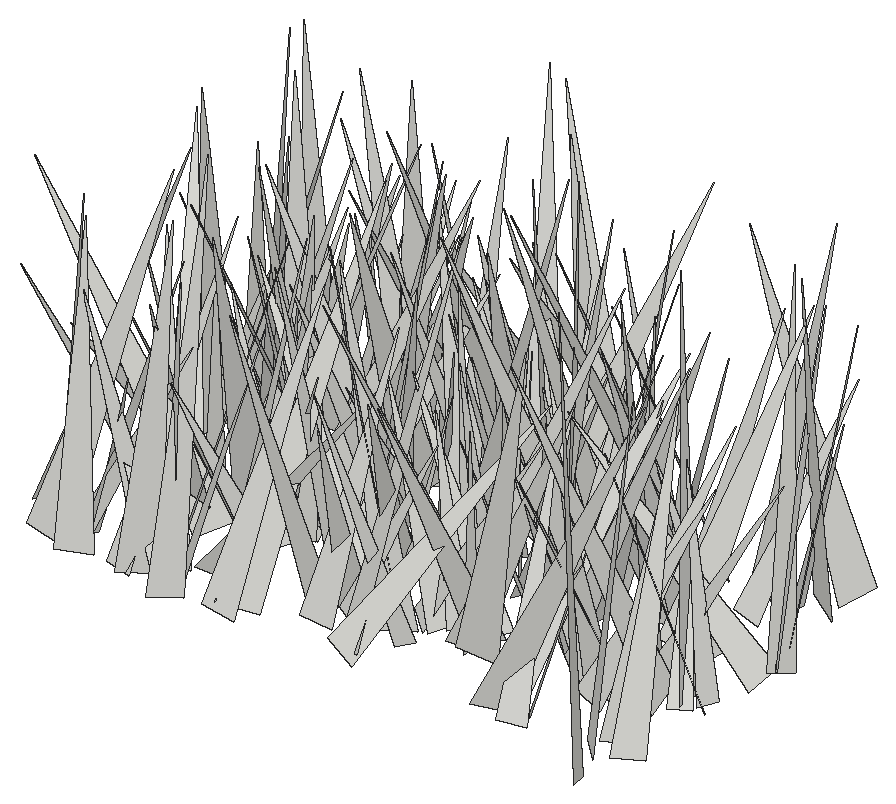
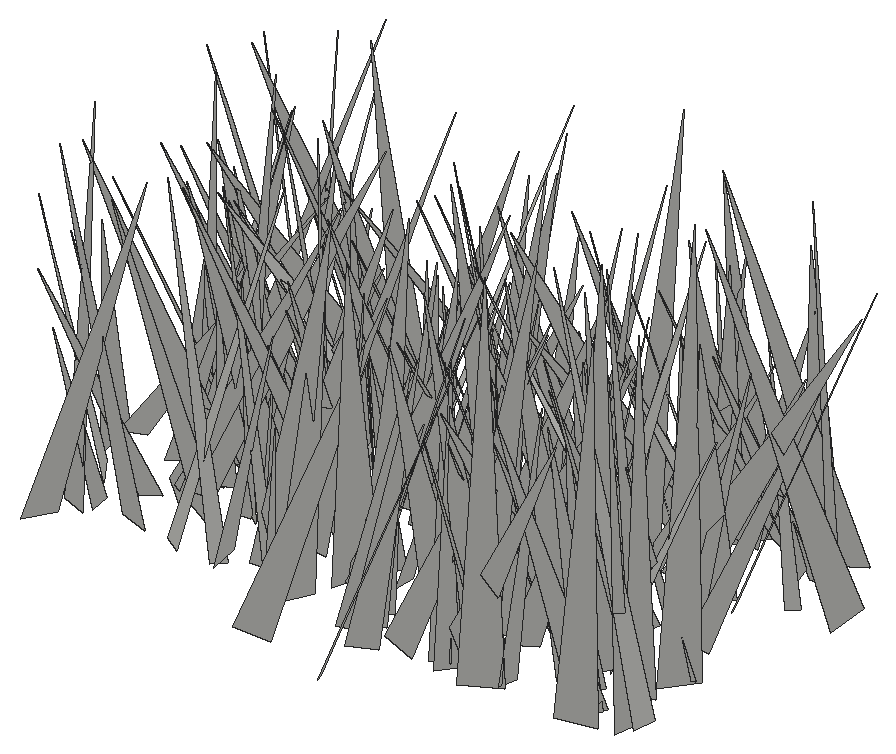
# SketchUp Ruby script. Lengths in inches.
U = 1.inch
M = Sketchup.active_model
def pt(a) = Geom::Point3d.new(a.map { |v| v * U })
def face(e, loops, mat)
  f = e.add_face(loops[0].map { |a| pt(a) })
  loops[1..].each { |l| e.add_face(l.map { |a| pt(a) }).erase! }
  f.material = f.back_material = mat if mat
  f
end
# faces: each face lists its corners as indices into pts; further lists are holes
def faces(e, pts, list, mat = nil) = list.each { |f| face(e, (f[0].is_a?(Array) ? f : [f]).map { |l| l.map { |i| pts[i] } }, mat) }
# xy, xz, yz: faces in a plane at the given z, y or x. An outline is a flat list of corners, or four numbers for a rectangle; further outlines are holes
def ring(l) = l.size == 4 ? [[l[0], l[1]], [l[2], l[1]], [l[2], l[3]], [l[0], l[3]]] : l.each_slice(2).to_a
def flat(e, list, mat, &to3) = list.each { |f| face(e, (f[0].is_a?(Array) ? f : [f]).map { |l| ring(l).map { |u, v| to3.(u, v) } }, mat) }
def xy(e, z, list, mat = nil) = flat(e, list, mat) { |x, y| [x, y, z] }
def xz(e, y, list, mat = nil) = flat(e, list, mat) { |x, z| [x, y, z] }
def yz(e, x, list, mat = nil) = flat(e, list, mat) { |y, z| [x, y, z] }
def lines(e, pts, list) = list.each { |a, b| e.add_line(pt(pts[a]), pt(pts[b])) }
# prism: a flat outline (further loops are holes) pulled along v
def prism(e, loops, v, mat = nil)
  f = face(e, loops, mat); d = Geom::Vector3d.new(v.map { |x| x * U })
  f.pushpull(f.normal.samedirection?(d) ? d.length : -d.length)
end
def box(e, o, s, mat = nil) = prism(e, [[o, [o[0] + s[0], o[1], o[2]], [o[0] + s[0], o[1] + s[1], o[2]], [o[0], o[1] + s[1], o[2]]]], [0, 0, s[2]], mat)
def at(x, y, z, deg = 0) = Geom::Transformation.translation(pt([x, y, z])) * Geom::Transformation.rotation(ORIGIN, Z_AXIS, deg.degrees)
def axes(o, x, y, z) = Geom::Transformation.new([*x, 0, *y, 0, *z, 0, *pt(o).to_a, 1])
def part(name) = M.definitions.add(name)
# library, detail: a bought-in or finely detailed component or shape, given as its bounding box
def library(name, o, s) = part(name).tap { |d| box(d.entities, o, s) }
def detail(e, o, s) = box(e.add_group.entities, o, s)
def put(e, d, t, mat = nil) = e.add_instance(d, t).tap { |i| i.material = mat if mat }
def group(e, t, mat = nil) = e.add_group.tap { |g| g.transformation = t; g.material = mat if mat }.entities
root = M.entities
c1 = part("fur_instance\#9")
p = [[0.8125,0,1.79],[0.67,-0.02,1.48],[0,-0.11,0],[0,0.11,0]]
faces(c1.entities,p,[[0,1,2,3]])
put(root,c1,axes([504.1,56.19,-21.86],[-7.32928,-2.99407,2.48715],[-3.76161,6.81126,-2.88543],[1.00033,3.67572,7.37273]))
put(root,c1,axes([480.44,57.9,-21.86],[-2.28357,5.70644,2.33564],[6.0895,2.47813,-0.10083],[0.96778,-2.12809,6.14557]))
put(root,c1,axes([483.11,58.11,-21.86],[4.75602,-4.66812,2.75377],[-5.20371,-4.95731,0.58378],[-1.51526,2.37234,6.63855]))
put(root,c1,axes([478.87,59.24,-21.86],[6.37942,2.61315,2.43113],[3.05762,-6.56979,-0.96169],[-1.84118,-1.85616,6.82648]))
put(root,c1,axes([483.21,58.84,-21.66],[0.69074,-4.72184,2.34998],[-4.89788,-1.45354,-1.48096],[-1.95676,1.97148,4.53648]))
put(root,c1,axes([503.06,58.16,-21.86],[4.54729,4.68314,2.12923],[4.88324,-4.82336,0.17985],[-1.61844,-1.39522,6.52513]))
put(root,c1,axes([484.17,58.3,-21.66],[-2.33068,3.85921,0.35584],[3.66264,2.05758,1.6744],[-1.26695,-1.15111,4.18592]))
put(root,c1,axes([479.25,57.9,-21.66],[0.24663,7.62872,2.41582],[7.70784,0.42293,-2.12242],[2.15005,-2.39126,7.33168]))
put(root,c1,axes([484.18,58.44,-21.86],[3.06348,4.37723,2.06786],[4.6001,-3.39453,0.37061],[-1.50841,-1.46222,5.32989]))
put(root,c1,axes([498.79,57.98,-21.66],[5.79439,-3.93356,1.43708],[-4.17619,-5.2444,2.48372],[0.31237,2.85246,6.54821]))
put(root,c1,axes([489.16,60.53,-21.86],[-5.96376,-1.66281,1.60864],[-1.32131,6.09893,1.40577],[1.89916,-0.97833,6.02952]))
put(root,c1,axes([490.28,61.08,-21.86],[3.42227,-3.49613,0.30492],[-3.40506,-3.41104,-0.89344],[-0.84941,-0.41195,4.81005]))
put(root,c1,axes([487.02,57.62,-21.86],[0.10942,6.44965,1.02032],[6.44115,0.06102,-1.07648],[1.07264,-1.02435,6.36012]))
put(root,c1,axes([495.81,61.57,-21.66],[2.24091,-5.47361,0.67385],[-5.23088,-2.33999,-1.61199],[-1.7471,-0.01469,5.69066]))
put(root,c1,axes([479.77,59.16,-21.86],[2.82226,4.09729,0.68802],[3.94816,-2.38599,-1.98631],[1.29353,-1.65697,4.56152]))
put(root,c1,axes([499.8,57.86,-21.86],[-1.60174,4.9541,0.61833],[4.97114,1.64265,-0.28364],[0.46172,-0.4996,5.19887]))
put(root,c1,axes([479.1,61.22,-21.86],[4.69242,0.16576,0.10905],[0.19618,-4.2622,-1.96297],[-0.02968,-1.96577,4.26532]))
put(root,c1,axes([484.67,58.49,-21.86],[3.7464,3.46532,0.67043],[3.46985,-3.79505,0.22613],[-0.64655,-0.28736,5.09832]))
put(root,c1,axes([499.99,63.17,-21.66],[-3.50557,-5.51536,0.11612],[-4.95597,3.20905,2.80393],[2.42302,-1.41579,5.90306]))
put(root,c1,axes([496.09,60.58,-21.66],[2.2039,-6.87435,1.74953],[-7.02125,-1.85328,1.56272],[1.00974,2.1174,7.04782]))
put(root,c1,axes([493.7,59.63,-21.66],[-0.77186,4.35622,1.72795],[4.2436,-0.09339,2.13104],[-1.98854,-1.8902,3.87699]))
put(root,c1,axes([503.06,62.18,-21.66],[-7.42684,-1.75978,1.28146],[-1.36577,7.3143,2.12899],[1.69519,-1.81689,7.32954]))
put(root,c1,axes([484.9,62.6,-21.66],[7.37439,-3.31849,1.28024],[-2.90244,-7.31769,-2.24953],[-2.05603,-1.57231,7.76747]))
put(root,c1,axes([480.76,62.38,-21.86],[-5.31145,-3.30369,0.30508],[-3.10318,5.15062,1.7494],[1.17379,-1.33255,6.00546]))
put(root,c1,axes([483.85,58.97,-21.86],[-3.36286,5.21282,1.50099],[5.38655,3.41774,0.19865],[0.64152,-1.37145,6.20023]))
put(root,c1,axes([497.47,60.89,-21.86],[3.7363,2.07589,0.22504],[1.88074,-3.14536,-2.2112],[0.90706,-2.02911,3.65784]))
put(root,c1,axes([492.25,57.82,-21.66],[0.90469,6.24799,0.05202],[5.52251,-0.775,-2.9597],[2.92267,-0.46962,5.57638]))
put(root,c1,axes([485.13,57.0625,-21.66],[-7.34828,2.49323,1.09592],[2.03506,7.1224,-2.5582],[1.80991,2.11416,7.32591]))
put(root,c1,axes([482.32,62.46,-21.86],[0.60186,-6.09784,0.10298],[-6.0697,-0.58883,0.60707],[0.59415,0.16161,6.09732]))
put(root,c1,axes([485.96,61.68,-21.86],[-4.12735,0.23871,1.0618],[0.66209,3.85593,1.70672],[0.86374,-1.81501,3.76552]))
put(root,c1,axes([490.9,59.92,-21.66],[1.63148,3.88333,0.8996],[3.80186,-1.22375,-1.61232],[1.19808,-1.40479,3.89132]))
put(root,c1,axes([490.08,59.21,-21.86],[-0.68675,5.73435,1.62653],[5.78722,1.03346,-1.2],[1.42703,-1.4315,5.64928]))
put(root,c1,axes([490.99,63,-21.66],[5.45875,-2.61976,0.1584],[-2.41646,-5.15945,-2.05595],[-1.02417,-1.78972,5.6951]))
put(root,c1,axes([494.09,63.34,-21.66],[-5.79035,-4.99721,0.36352],[-4.82955,5.71454,1.62848],[1.33407,-1.00217,7.47317]))
put(root,c1,axes([500.6,61.71,-21.86],[4.51587,-1.82573,1.61231],[-1.49442,-4.75873,-1.20297],[-1.92343,-0.58918,4.72009]))
put(root,c1,axes([482.36,57.92,-21.86],[2.22729,6.28936,0.04999],[6.2767,-2.22605,0.40869],[-0.40191,0.08939,6.65956]))
put(root,c1,axes([492.16,61.09,-21.86],[4.02018,4.80904,4.066],[5.52928,-5.00439,0.45193],[-3.01434,-2.76593,6.25176]))
put(root,c1,axes([495.41,60.79,-21.66],[3.73995,-4.97965,1.07609],[-4.97131,-3.27521,2.12161],[1.114,2.10195,5.85517]))
put(root,c1,axes([486.33,59.02,-21.86],[4.06792,5.19434,1.22411],[5.14399,-4.22635,0.83955],[-1.42088,-0.42943,6.54403]))
put(root,c1,axes([492.65,60.54,-21.86],[0.55965,-6.1533,3.26603],[-6.71098,-1.35523,-1.40332],[-1.86889,3.02383,6.01722]))
put(root,c1,axes([480.29,58.99,-21.66],[4.99403,0.89918,1.35491],[0.3935,-4.91429,1.81096],[-1.5778,1.62046,4.74018]))
put(root,c1,axes([485.15,59.38,-21.66],[4.61387,-2.10989,0.31356],[-1.93342,-3.82099,2.73855],[0.90102,2.60502,4.2708]))
put(root,c1,axes([504.49,58.43,-21.86],[-5.42402,3.35952,0.54018],[3.08821,5.28712,-1.87283],[1.42868,1.32596,6.09909]))
put(root,c1,axes([498.83,62.82,-21.86],[1.2889,-4.23263,0.01136],[-4.22076,-1.28617,-0.32791],[-0.31699,-0.08469,4.41236]))
put(root,c1,axes([503.36,59.02,-21.86],[-4.3486,2.21974,0.80785],[1.83051,4.23636,-1.78683],[1.49303,1.27131,4.54366]))
put(root,c1,axes([495.49,61.08,-21.86],[-3.94466,-0.14605,1.57067],[-0.23954,4.23653,-0.20765],[1.55915,0.28136,3.94189]))
put(root,c1,axes([504.04,63.01,-21.86],[-3.65311,-4.50937,0.62916],[-4.48426,3.70309,0.50402],[0.78847,0.16789,5.78149]))
put(root,c1,axes([484.62,62.13,-21.66],[-2.52034,-4.28654,0.32351],[-4.12689,2.30776,-1.57296],[-1.20326,1.06349,4.71724]))
put(root,c1,axes([500.8125,60.82,-21.86],[0.87918,5.14411,1.43079],[4.85097,-0.16366,-2.39235],[2.23095,-1.67133,4.63805]))
put(root,c1,axes([500.65,61.4,-21.86],[-0.27177,-3.75184,1.87256],[-3.70908,-0.66019,-1.86105],[-1.95589,1.77327,3.26904]))
put(root,c1,axes([492.36,58.14,-21.66],[3.62911,6.60842,0.2466],[6.35712,-3.56375,1.94657],[-1.82181,0.72867,7.28371]))
put(root,c1,axes([477.17,60.625,-21.86],[7.79072,-0.23447,0.87822],[-0.35324,-7.76347,1.06082],[-0.83754,1.09323,7.72172]))
put(root,c1,axes([488.57,62.52,-21.86],[-6.02473,-0.71032,1.74625],[-0.51818,6.24626,0.75302],[1.81257,-0.57532,6.01954]))
put(root,c1,axes([483.25,62.12,-21.86],[-4.16636,5.9481,1.52453],[5.74666,3.12806,3.50054],[-2.16332,-3.14611,6.36276]))
put(root,c1,axes([493.76,61.55,-21.86],[-4.44101,1.77663,0.66677],[1.83519,4.45274,0.3588],[0.48276,-0.58331,4.76973]))
put(root,c1,axes([498.64,58.67,-21.86],[-2.65177,6.66161,0.65253],[5.97681,2.67255,-2.995],[3.01341,0.56142,6.51452]))
put(root,c1,axes([492.76,61.55,-21.86],[2.95433,4.07724,0.35212],[3.82019,-2.59183,-2.04072],[1.46767,-1.46099,4.60298]))
put(root,c1,axes([485.59,62.22,-21.86],[4.21997,-0.6182,0.41958],[-0.60999,-4.24047,-0.11271],[-0.43142,-0.05127,4.26352]))
put(root,c1,axes([496.74,62.95,-21.86],[5.27182,0.13194,1.25121],[0.40362,-5.28245,-1.14356],[-1.19165,-1.2055,5.14798]))
put(root,c1,axes([487.34,58.3,-21.86],[-5.76444,5.45156,1.05869],[4.71185,5.60881,-3.22628],[2.93919,1.70025,7.24841]))
put(root,c1,axes([494.29,61.92,-21.86],[-2.34318,3.21724,1.23905],[3.43189,2.31946,0.46753],[0.3286,-1.2829,3.95253]))
put(root,c1,axes([483.73,59.32,-21.86],[4.88269,3.53574,0.69101],[3.04894,-4.67553,2.3797],[-1.91908,1.56767,5.53887]))
put(root,c1,axes([498.39,62.54,-21.66],[4.54413,5.8348,1.67226],[5.93472,-3.83302,-2.75273],[1.27295,-2.95864,6.86415]))
put(root,c1,axes([479.79,65.66,-21.66],[4.40481,-2.70951,0.82389],[-1.71706,-3.76665,-3.20728],[-2.2521,-2.42766,4.05674]))
put(root,c1,axes([495.58,62.41,-21.86],[-3.16425,3.77948,0.90882],[3.82647,2.82214,1.58634],[-0.68447,-1.69527,4.66695]))
put(root,c1,axes([501.33,61.07,-21.66],[0.65579,5.75921,0.77226],[5.58682,-0.41126,-1.67728],[1.5976,-0.92592,5.54845]))
put(root,c1,axes([482.58,63.01,-21.86],[4.66089,-0.94094,1.87831],[-0.93791,-5.02216,-0.1885],[-1.87983,0.17273,4.75118]))
put(root,c1,axes([491.84,61.29,-21.86],[2.15657,3.40289,0.33157],[3.29952,-2.17412,0.8525],[-0.89598,0.18416,3.93747]))
put(root,c1,axes([485.83,62.66,-21.86],[-4.37438,2.14658,0.79892],[2.22863,4.38643,0.41683],[0.52851,-0.72986,4.85482]))
put(root,c1,axes([498.67,59.9375,-21.86],[4.76717,4.34009,0.09976],[4.0907,-4.54047,2.05487],[-1.45344,1.45601,6.11063]))
put(root,c1,axes([496.86,63.15,-21.86],[-3.19994,-2.12817,0.10035],[-2.08753,3.09569,-0.91527],[-0.42587,0.81635,3.73243]))
put(root,c1,axes([494.23,61.85,-21.66],[3.12045,6.97557,0.92804],[6.87353,-2.80376,-2.03727],[1.5081,-1.6545,7.36514]))
put(root,c1,axes([500.16,58.4375,-21.66],[5.94606,5.36025,0.59468],[4.2161,-5.17199,4.4628],[-3.36309,2.9933,6.64615]))
put(root,c1,axes([486.17,63.41,-21.86],[2.50338,-2.82714,1.30611],[-3.05988,-2.54469,0.35667],[-0.57944,1.22368,3.75931]))
put(root,c1,axes([481.11,64.24,-21.86],[-1.67954,-4.60165,1.09216],[-4.72861,1.65608,-0.29411],[0.09072,1.12742,4.88974]))
put(root,c1,axes([486.01,64.34,-21.86],[-1.02707,-3.52995,0.46815],[-3.49734,0.90838,-0.82343],[-0.66956,0.66999,3.58293]))
put(root,c1,axes([493.96,63.96,-21.86],[0.28904,-4.61969,1.68996],[-4.89331,-0.44312,-0.3744],[-0.50298,1.65624,4.61355]))
put(root,c1,axes([503.72,62.26,-21.86],[-2.57238,2.98987,0.10946],[2.97729,2.57237,-0.29516],[0.29502,0.10983,3.93311]))
put(root,c1,axes([490.69,65.67,-21.86],[1.56687,-4.2825,0.24372],[-4.04586,-1.5617,-1.43053],[-1.42486,-0.27491,4.32996]))
put(root,c1,axes([489.04,62.95,-21.66],[-3.06534,4.86368,0.18481],[4.51167,2.75744,2.26433],[-1.82603,-1.35165,5.28436]))
put(root,c1,axes([504.25,63.14,-21.86],[-4.36363,0.98227,0.81119],[0.91976,4.432,-0.41906],[0.88144,0.23814,4.45315]))
put(root,c1,axes([489.42,62.61,-21.86],[5.30824,4.83924,1.79848],[4.88732,-5.54151,0.48577],[-1.6634,-0.83881,7.16657]))
put(root,c1,axes([489.14,65.14,-21.86],[0.61294,-5.47928,1.38132],[-5.30961,-1.0339,-1.7451],[-1.93355,1.10218,5.22999]))
put(root,c1,axes([494.61,62.23,-21.66],[1.00631,5.78428,1.17144],[5.41169,-1.37849,2.15781],[-2.35451,-0.6962,5.46025]))
put(root,c1,axes([504.66,65.7,-21.86],[-5.96221,1.49508,0.02596],[1.36332,5.39133,2.61894],[-0.61423,-2.54602,5.56097]))
put(root,c1,axes([501.52,63.6875,-21.86],[3.29682,4.04593,0.27696],[3.82738,-2.98619,-1.93627],[1.34069,-1.42422,4.84659]))
put(root,c1,axes([503.54,63,-21.86],[-7.33304,-1.55705,2.53328],[-2.07568,7.50758,-1.39398],[2.1292,1.95633,7.36578]))
put(root,c1,axes([496.47,66.49,-21.66],[-7.7703,-1.5883,1.42664],[-1.2052,7.70803,2.01725],[1.76224,-1.7318,7.67014]))
put(root,c1,axes([499.97,65.46,-21.86],[-3.27673,-6.38483,2.25273],[-6.55108,3.62196,0.73666],[1.71005,1.64109,7.13865]))
put(root,c1,axes([488.47,65.77,-21.86],[6.1777,-0.38175,1.16241],[-0.13775,-6.16226,-1.29169],[-1.21571,-1.24165,6.0532]))
put(root,c1,axes([500.65,66.79,-21.86],[1.25653,-6.81976,0.6894],[-6.81087,-1.32116,-0.65555],[-0.77223,0.55558,6.90349]))
put(root,c1,axes([481.75,62.23,-21.86],[-3.35316,6.39569,0.22234],[6.39729,3.34326,0.30873],[-0.17041,-0.34016,7.2148]))
put(root,c1,axes([483.33,65.99,-21.66],[0.81031,-5.69395,0.84212],[-5.55553,-0.55126,1.61834],[1.50543,1.03047,5.51893]))
put(root,c1,axes([484.76,65.59,-21.86],[-4.52954,-3.25843,1.35312],[-3.24257,4.71245,0.49358],[1.39071,0.3748,5.55792]))
put(root,c1,axes([482.9375,68.11,-21.86],[-3.5223,-6.70382,0.02091],[-6.50166,3.42181,1.83516],[1.63401,-0.83562,7.34711]))
put(root,c1,axes([497.63,65.5,-21.86],[5.75538,-1.33671,0.29214],[-1.31847,-5.75568,-0.36093],[-0.36579,-0.28603,5.89753]))
put(root,c1,axes([488.43,63.11,-21.86],[-0.08905,4.06249,0.07241],[4.03019,0.09752,-0.5148],[0.51634,-0.06053,4.03072]))
put(root,c1,axes([484.27,66.37,-21.66],[6.50516,0.09741,3.11354],[0.81371,-7.01185,-1.48071],[-3.00691,-1.68675,6.33514]))
put(root,c1,axes([488.26,64.5,-21.86],[6.38411,4.40631,2.11358],[4.61615,-6.57865,-0.22824],[-1.60436,-1.39477,7.75373]))
put(root,c1,axes([489.65,66.72,-21.86],[4.97524,0.71585,1.07536],[1.04452,-4.74693,-1.67259],[-0.76015,-1.83742,4.74004]))
put(root,c1,axes([487.48,68.32,-21.66],[7.10031,-2.91459,1.55919],[-2.29482,-7.00551,-2.64516],[-2.37902,-1.94118,7.20502]))
put(root,c1,axes([502.35,66.26,-21.86],[-3.89042,0.9571,1.21715],[1.27935,3.84105,1.06884],[0.87221,-1.36496,3.86121]))
put(root,c1,axes([485.47,64.31,-21.86],[2.59444,7.48207,1.23534],[7.31718,-2.12705,-2.48457],[1.99156,-1.93206,7.51927]))
put(root,c1,axes([492.47,67.1875,-21.86],[1.67975,-3.93598,0.16611],[-3.93538,-1.66827,0.26597],[0.17974,0.25696,4.27115]))
put(root,c1,axes([492.36,64.86,-21.86],[-1.21025,6.4146,1.42422],[6.45546,0.89059,1.47445],[-1.22575,-1.64315,6.35907]))
put(root,c1,axes([478.85,67.82,-21.86],[7.55718,-3.05255,1.8054],[-2.7949,-7.74218,-1.39129],[-2.18313,-0.65505,8.03077]))
put(root,c1,axes([484.01,63.5,-21.86],[5.80303,5.01805,0.27093],[4.96083,-5.78629,0.91567],[-0.80277,0.51711,7.61693]))
put(root,c1,axes([499.78,66.62,-21.86],[0.85171,-3.4207,0.8533],[-3.50883,-0.73716,0.54719],[0.34265,0.95401,3.48241]))
put(root,c1,axes([497.82,68.2,-21.66],[3.38324,-1.277,0.34003],[-0.90165,-2.91389,-1.97203],[-0.96612,-1.75247,3.03119]))
put(root,c1,axes([493.62,66.04,-21.86],[3.14318,2.78213,1.66083],[2.96777,-3.40061,0.07991],[-1.30037,-1.03624,4.19683]))
put(root,c1,axes([495.13,65.65,-21.86],[4.37398,5.97616,2.1686],[6.29129,-4.44766,-0.43255],[-0.91492,-2.01317,7.39318]))
put(root,c1,axes([494.39,65.0625,-21.86],[4.56042,0.58445,0.815],[0.35248,-4.48653,1.24501],[-0.93891,1.15443,4.42595]))
put(root,c1,axes([492.39,67.45,-21.86],[-4.23671,-2.59002,0.97553],[-2.55905,4.34534,0.42292],[1.0541,0.13924,4.94763]))
put(root,c1,axes([496.08,65.73,-21.86],[-6.60957,-3.13791,3.29203],[-3.79035,7.01015,-0.92809],[2.51341,2.31982,7.25752]))
put(root,c1,axes([488.46,65.34,-21.66],[-5.41908,-0.82486,1.13145],[-1.12996,5.24719,-1.58656],[0.82691,1.76453,5.24687]))
put(root,c1,axes([490.73,68.125,-21.86],[-5.81258,-1.56867,1.18702],[-1.32265,5.85738,1.26392],[1.45614,-0.94136,5.88637]))
put(root,c1,axes([492.32,64.11,-21.86],[7.12046,1.58475,2.39098],[0.70942,-7.17277,2.64146],[-2.77938,2.22916,6.79964]))
put(root,c1,axes([495.375,67.24,-21.86],[-0.82021,3.34867,1.94688],[3.86928,0.61559,0.57127],[-0.18046,-2.02092,3.4]))
put(root,c1,axes([500.09,68.32,-21.86],[-2.49506,-7.82927,1.12782],[-7.54738,2.00233,-2.79687],[-2.3678,1.86761,7.7266]))
put(root,c1,axes([486.38,65.64,-21.86],[1.81357,5.35205,0.20733],[5.12174,-1.66889,-1.72019],[1.56691,-0.73948,5.38279]))
put(root,c1,axes([481.94,65.89,-21.66],[4.14579,-2.60609,2.17076],[-3.31381,-3.84297,1.71517],[-0.72292,2.67047,4.58667]))
put(root,c1,axes([485.58,68.54,-21.86],[5.39011,-5.98506,0.75501],[-6.02641,-5.29691,1.03406],[0.27067,1.25142,7.9878]))
put(root,c1,axes([500.95,65.53,-21.86],[-0.63507,6.95916,1.46669],[6.78735,1.03289,-1.962],[2.12438,-1.21968,6.70699]))
put(root,c1,axes([496.51,67.33,-21.86],[5.13759,-3.83835,0.8309],[-3.9202,-4.93031,1.46363],[0.23526,1.66651,6.24384]))
put(root,c1,axes([496.17,65.55,-21.86],[0.66695,4.37993,0.08385],[4.36286,-0.67176,0.3871],[-0.39533,-0.02429,4.41347]))
put(root,c1,axes([487.66,67.42,-21.86],[-2.49049,-3.07283,1.62396],[-3.33154,2.67981,-0.03854],[0.99012,1.28779,3.95516]))
put(root,c1,axes([481.58,68.15,-21.86],[3.73813,0.01426,0.67221],[0.17612,-3.68545,-0.90117],[-0.64889,-0.91811,3.62791]))
put(root,c1,axes([478.83,67.34,-21.86],[-0.2038,-3.57727,1.86557],[-3.68837,0.92217,1.36537],[1.63497,1.63446,3.31273]))
put(root,c1,axes([481.68,68.13,-21.86],[-3.75562,-3.58045,0.3486],[-3.58145,3.67402,-0.84892],[-0.33818,0.85312,5.11895]))
put(root,c1,axes([491.55,67.61,-21.86],[1.31397,-3.56018,1.31098],[-3.78942,-1.16427,0.63629],[0.18405,1.44556,3.7412]))
put(root,c1,axes([482.19,66.04,-21.66],[-7.10447,-2.39928,3.44832],[-3.25719,7.42464,-1.54476],[2.65295,2.69055,7.33783]))
put(root,c1,axes([500.8,68.17,-21.86],[-4.44374,-5.75342,0.61079],[-5.6055,4.0905,-2.25122],[-1.43294,1.84058,6.91236]))
put(root,c1,axes([486.62,68.15,-21.86],[3.50873,2.55931,1.93983],[3.03472,-3.58228,-0.76287],[-1.05048,-1.80039,4.27543]))
put(root,c1,axes([495.82,68.56,-21.66],[-1.13695,-6.80591,1.9758],[-6.92615,0.64332,-1.76957],[-1.50086,2.18691,6.66945]))
put(root,c1,axes([481.59,68.6875,-21.86],[3.84963,-3.94903,0.87916],[-4.01863,-3.87266,0.20133],[-0.4673,0.77142,5.51126]))
put(root,c1,axes([482.33,68.06,-21.86],[4.03772,-5.94106,3.0996],[-6.44975,-4.42725,-0.08397],[-1.8178,2.512,7.18278]))
put(root,c1,axes([490.3125,70.33,-21.86],[2.21636,-6.61774,0.25451],[-6.61771,-2.20273,0.35418],[0.25535,0.35358,6.97003]))
put(root,c1,axes([496.16,69.27,-21.86],[-2.04339,-2.88899,0.9747],[-2.5158,2.26047,1.42575],[1.7225,-0.12566,3.23866]))
put(root,c1,axes([494.73,65.73,-21.86],[-0.48607,6.36101,0.33267],[6.36907,0.48063,0.1158],[-0.09028,-0.34048,6.37851]))
put(root,c1,axes([479.46,69.23,-21.86],[0.11264,-6.37998,1.60761],[-6.5012,0.13924,1.0081],[1.01142,1.60553,6.30084]))
put(root,c1,axes([492.01,69.48,-21.86],[-2.55131,-7.67351,1.38924],[-7.65133,2.18082,-2.00574],[-1.50657,1.91917,7.83383]))
put(root,c1,axes([484.58,69.28,-21.66],[-5.48359,2.23586,1.70204],[2.68404,5.27249,1.72124],[0.83185,-2.27324,5.66623]))
put(root,c1,axes([484.99,67.45,-21.86],[3.70587,4.25797,0.60198],[4.28884,-3.60158,-0.92773],[0.31394,-1.06043,5.56805]))
put(root,c1,axes([497.92,67.63,-21.86],[2.53366,4.26731,1.78001],[4.34271,-2.89305,0.75426],[-1.5872,-1.10369,4.90515]))
put(root,c1,axes([484.93,66.3,-21.86],[-4.41851,1.16155,1.66424],[0.34777,4.36157,-2.12081],[1.99949,1.8082,4.04655]))
put(root,c1,axes([498.7,70.98,-21.86],[-4.09518,-5.32392,0.52178],[-5.17841,4.11019,1.29512],[1.34181,-0.38619,6.5907]))
put(root,c1,axes([481.69,69.83,-21.66],[3.71453,-6.09838,0.78607],[-6.05056,-3.46164,1.73599],[1.09493,1.55972,6.92635]))
put(root,c1,axes([486.46,67.35,-21.86],[1.13394,4.06883,0.24777],[4.07369,-1.14042,0.08414],[-0.14769,-0.216,4.22305]))
put(root,c1,axes([480.25,68.5,-21.86],[3.54049,4.95211,1.34575],[5.12044,-3.30078,-1.32493],[0.33991,-1.85767,5.94164]))
put(root,c1,axes([492.1,67.57,-21.66],[-6.74391,-2.32387,0.77011],[-2.44649,6.31426,-2.37034],[-0.09,2.49068,6.72772]))
put(root,c1,axes([496.625,71.03,-21.86],[6.71484,1.18998,0.43364],[1.2609,-6.06064,-2.89345],[0.11927,-2.92333,6.1752]))
put(root,c1,axes([493.99,67.27,-21.86],[-6.04222,-2.58238,2.07365],[-3.21518,5.60869,-2.38377],[0.79453,3.05796,6.1233]))
put(root,c1,axes([486.43,65.71,-21.66],[-4.56686,4.07542,0.09193],[3.68922,4.19072,-2.51023],[1.73411,1.8173,5.58247]))
put(root,c1,axes([486.96,69.03,-21.86],[1.79805,-6.87497,3.712],[-7.43664,-2.674,-1.35027],[-2.39594,3.14033,6.97674]))
put(root,c1,axes([504.51,66.375,-21.86],[3.51213,5.3509,1.08193],[4.75447,-3.63032,2.52063],[-2.68285,0.57134,5.88334]))
put(root,c1,axes([499.46,68.2,-21.86],[1.23681,5.98503,1.54047],[6.1022,-0.934,-1.27052],[0.97821,-1.7408,5.97797]))
put(root,c1,axes([504.84,66.48,-21.86],[-7.06937,0.92542,0.80535],[0.55425,6.6114,-2.73188],[1.09444,2.62944,6.58553]))
put(root,c1,axes([494.6,68.53,-21.66],[-1.73609,5.26171,0.91511],[5.1615,1.40586,1.70864],[-1.37182,-1.3693,5.27069]))
put(root,c1,axes([481.01,70.01,-21.86],[3.21186,-3.52218,0.8528],[-3.62385,-3.13,0.72104],[-0.02677,1.11644,4.71189]))
put(root,c1,axes([480.06,71.27,-21.86],[0.93957,-4.99379,0.05949],[-4.70596,-0.86502,1.71172],[1.67197,0.37157,4.78443]))
put(root,c1,axes([477.8125,71.03,-21.66],[8.03575,1.73258,0.69022],[1.85682,-7.7181,-2.24381],[-0.17451,-2.34107,7.90825]))
put(root,c1,axes([488.09,71.76,-21.86],[-1.10699,-6.38687,0.31821],[-6.26084,1.01671,-1.37367],[-1.30201,0.54128,6.33487]))
put(root,c1,axes([503.73,68.4,-21.86],[-4.45958,-2.36263,3.46386],[-3.3219,5.07642,-0.81428],[2.55838,2.47306,4.98064]))
put(root,c1,axes([503.09,70.93,-21.86],[-3.13728,-6.42445,2.27927],[-6.51063,3.56742,1.09378],[2.01998,1.52023,7.06539]))
put(root,c1,axes([492,69.18,-21.86],[-1.66543,4.2087,0.7623],[4.0491,1.28782,1.73616],[-1.37806,-1.30242,4.18002]))
put(root,c1,axes([492.68,68.1,-21.66],[1.48421,7.77893,1.22221],[7.56365,-1.06243,-2.42301],[2.19017,-1.60247,7.53948]))
put(root,c1,axes([484.43,71.35,-21.66],[3.61715,-5.66391,0.01487],[-5.50634,-3.51236,1.58351],[1.3268,0.86448,6.53117]))
put(root,c1,axes([486.34,71.6875,-21.86],[-0.53016,-5.209,0.61736],[-4.97847,0.69512,1.58982],[1.65216,0.4231,4.98871]))
put(root,c1,axes([489.72,67.49,-21.66],[-6.30964,2.41528,1.06239],[1.96226,6.1361,-2.29599],[1.76402,1.81341,6.35402]))
put(root,c1,axes([501.46,68.75,-21.86],[0.30593,5.01742,0.69432],[4.86404,-0.09691,-1.44288],[1.4134,-0.75252,4.8152]))
put(root,c1,axes([478.36,71.48,-21.86],[6.10646,0.88523,1.50787],[1.27518,-6.00248,-1.64024],[-1.19633,-1.87958,5.94829]))
put(root,c1,axes([483.56,71.375,-21.86],[4.6906,-0.13116,1.94102],[0.35682,-4.92253,-1.19491],[-1.91244,-1.24013,4.53774]))
put(root,c1,axes([485.85,71.95,-21.86],[5.31663,-1.02418,0.76649],[-0.77202,-5.18142,-1.56841],[-1.02002,-1.41668,5.18224]))
put(root,c1,axes([494.09,71.22,-21.86],[6.71325,2.37054,1.67819],[2.73448,-6.58312,-1.63968],[-0.97898,-2.13225,6.9281]))
put(root,c1,axes([489.67,71.19,-21.86],[3.16597,-2.82128,1.36449],[-2.73379,-3.43456,-0.75836],[-1.53229,0.2984,4.17228]))
put(root,c1,axes([490.14,71.81,-21.86],[2.45481,-4.16097,0.8917],[-4.06011,-2.59844,-0.9479],[-1.27449,0.26329,4.73722]))
put(root,c1,axes([502.45,70.32,-21.86],[3.57631,0.31891,0.97988],[0.16002,-3.66803,0.60973],[-1.01797,0.54376,3.53835]))
put(root,c1,axes([489.08,72.55,-21.86],[-3.71631,2.59474,2.95715],[3.6126,3.86147,1.15179],[1.55775,-2.76492,4.38373]))
put(root,c1,axes([492.19,68.95,-21.86],[-7.18499,4.19207,1.05141],[4.04317,7.24035,-1.23823],[1.52698,0.55406,8.22584]))
put(root,c1,axes([493.04,71.33,-21.86],[-6.55699,2.55506,2.62376],[2.8465,6.94107,0.35432],[2.30431,-1.30376,7.02829]))
put(root,c1,axes([500.72,70.6,-21.86],[3.30058,6.51639,2.13105],[6.85171,-3.21879,-0.76942],[-0.24255,-2.25268,7.26396]))
put(root,c1,axes([484.14,72.16,-21.86],[3.60415,-6.43604,2.10161],[-6.7075,-3.71823,0.11619],[-0.92131,1.89247,7.37557]))
put(root,c1,axes([496.67,70.67,-21.86],[-5.51822,-0.21879,0.79161],[-0.32668,5.51842,-0.75206],[0.75352,0.79022,5.4711]))
put(root,c1,axes([492.41,74.47,-21.66],[3.27442,-5.47757,0.11686],[-5.10679,-3.10069,-2.24625],[-1.98447,-1.05885,5.97327]))
put(root,c1,axes([494.57,70.53,-21.66],[-3.07753,7.46975,2.03134],[7.70521,2.74591,1.57617],[-0.74375,-2.46119,7.92363]))
put(root,c1,axes([479.97,71.25,-21.86],[2.95683,-4.48742,1.40063],[-4.613,-2.45121,1.88504],[0.90496,2.16707,5.03253]))
put(root,c1,axes([488.88,75.14,-21.86],[-5.64756,-4.03637,0.24701],[-3.60758,5.22048,2.82493],[1.82721,-2.16853,6.3409]))
put(root,c1,axes([503.57,72.26,-21.86],[-7.04891,1.70289,1.4017],[1.92518,7.04086,1.12767],[1.07622,-1.44158,7.16347]))
put(root,c1,axes([494.25,71.1875,-21.86],[-3.53666,-0.44387,1.07965],[-0.6619,3.59984,-0.68824],[0.96154,0.84544,3.49732]))
put(root,c1,axes([486.01,71.17,-21.66],[-1.67581,5.69721,1.32161],[5.39716,0.9769,2.63242],[-2.25291,-1.89755,5.32325]))
put(root,c1,axes([479.98,72.11,-21.86],[1.68119,-6.78383,2.85706],[-7.30642,-1.89388,-0.19753],[-0.89411,2.72073,6.98625]))
put(root,c1,axes([485.03,70.6875,-21.86],[2.64907,4.14771,0.84835],[4.17625,-2.72433,0.27885],[-0.69438,-0.56151,4.91358]))
